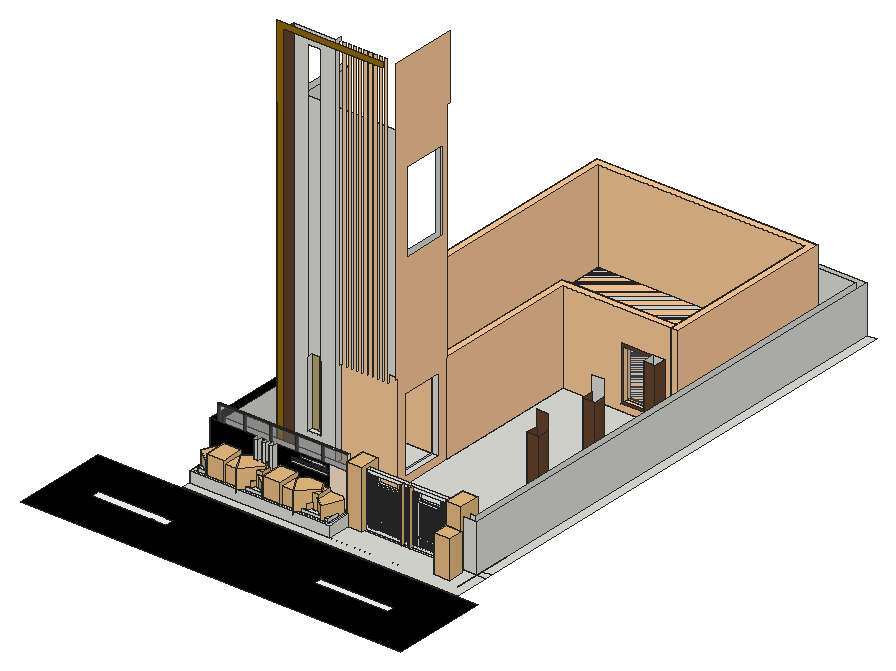
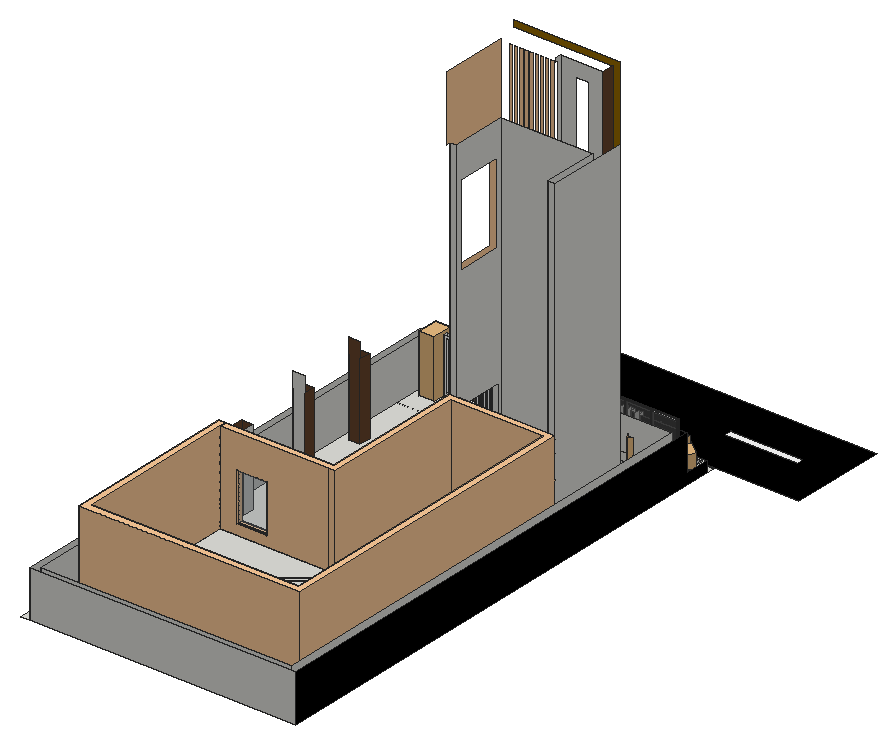
# SketchUp Ruby script. Lengths in inches.
U = 1.inch
M = Sketchup.active_model
def pt(a) = Geom::Point3d.new(a.map { |v| v * U })
def face(e, loops, mat)
  f = e.add_face(loops[0].map { |a| pt(a) })
  loops[1..].each { |l| e.add_face(l.map { |a| pt(a) }).erase! }
  f.material = f.back_material = mat if mat
  f
end
# faces: each face lists its corners as indices into pts; further lists are holes
def faces(e, pts, list, mat = nil) = list.each { |f| face(e, (f[0].is_a?(Array) ? f : [f]).map { |l| l.map { |i| pts[i] } }, mat) }
# xy, xz, yz: faces in a plane at the given z, y or x. An outline is a flat list of corners, or four numbers for a rectangle; further outlines are holes
def ring(l) = l.size == 4 ? [[l[0], l[1]], [l[2], l[1]], [l[2], l[3]], [l[0], l[3]]] : l.each_slice(2).to_a
def flat(e, list, mat, &to3) = list.each { |f| face(e, (f[0].is_a?(Array) ? f : [f]).map { |l| ring(l).map { |u, v| to3.(u, v) } }, mat) }
def xy(e, z, list, mat = nil) = flat(e, list, mat) { |x, y| [x, y, z] }
def xz(e, y, list, mat = nil) = flat(e, list, mat) { |x, z| [x, y, z] }
def yz(e, x, list, mat = nil) = flat(e, list, mat) { |y, z| [x, y, z] }
def lines(e, pts, list) = list.each { |a, b| e.add_line(pt(pts[a]), pt(pts[b])) }
# prism: a flat outline (further loops are holes) pulled along v
def prism(e, loops, v, mat = nil)
  f = face(e, loops, mat); d = Geom::Vector3d.new(v.map { |x| x * U })
  f.pushpull(f.normal.samedirection?(d) ? d.length : -d.length)
end
def box(e, o, s, mat = nil) = prism(e, [[o, [o[0] + s[0], o[1], o[2]], [o[0] + s[0], o[1] + s[1], o[2]], [o[0], o[1] + s[1], o[2]]]], [0, 0, s[2]], mat)
def at(x, y, z, deg = 0) = Geom::Transformation.translation(pt([x, y, z])) * Geom::Transformation.rotation(ORIGIN, Z_AXIS, deg.degrees)
def axes(o, x, y, z) = Geom::Transformation.new([*x, 0, *y, 0, *z, 0, *pt(o).to_a, 1])
def part(name) = M.definitions.add(name)
# library, detail: a bought-in or finely detailed component or shape, given as its bounding box
def library(name, o, s) = part(name).tap { |d| box(d.entities, o, s) }
def detail(e, o, s) = box(e.add_group.entities, o, s)
def put(e, d, t, mat = nil) = e.add_instance(d, t).tap { |i| i.material = mat if mat }
def group(e, t, mat = nil) = e.add_group.tap { |g| g.transformation = t; g.material = mat if mat }.entities
root = M.entities
M.materials.add("Asphalt_06_1K").color = [0, 0, 0]
M.materials.add("C01_Vanilla_Cream").color = [255, 230, 206]
M.materials.add("C02_Golden_Beige").color = [255, 205, 155]
M.materials.add("D07_Ochre_Flame").color = [153, 107, 0]
M.materials.add("Glass_Basic_01").color = [161, 173, 186]
M.materials["Glass_Basic_01"].alpha = 0.25
M.materials.add("Glass_Mirror_01").color = [185, 168, 118]
M.materials.add("M00_Soft_Cloud").color = [255, 255, 255]
M.materials.add("M09_Shadow_Night").color = [0, 0, 0]
M.materials.add("Material__1").color = [95, 70, 46]
M.materials.add("Wood_Veneer_15_1K").color = [103, 69, 45]
M.materials.add("[Color M00]").color = [255, 255, 255]
M.materials.add("[Color_000]").color = [255, 255, 255]
M.materials.add("[Color_C20]").color = [102, 91, 81]
M.materials.add("[Translucent Glass Gray]").color = [128, 128, 128]
M.materials["[Translucent Glass Gray]"].alpha = 0.29
c1 = library("Gate pillar",[0,0,0],[97.06,71.13,326.45])
c2 = library("Group_2",[-1.28,-0.39,0],[21.22,20.51,48.44])
c3 = library("Gate pull handle",[-0.01,0,0],[1.26,2.875,48])
c4 = part("Gate slat")
xy(c4.entities,0,[[0.39,114.16,6.3,114.17]])
xy(c4.entities,0,[[0.39,0,6.3,114.16]],"[Color_C20]")
xy(c4.entities,0.39,[[0.39,0,0.79,114.17],[0.98,0,2.07,114.17],[2.36,0,3.2,114.17],[3.59,0,4.37,114.17],[4.56,0,5.71,114.17],
  [5.91,0,6.3,114.17]],"[Color_C20]")
xy(c4.entities,0.79,[[0.39,0,0.79,114.17],[0.98,0,2.07,114.17],[2.36,0,3.2,114.17],[3.59,0,4.37,114.17],[4.56,0,5.71,114.17],
  [5.91,0,6.3,114.17]],"[Color_C20]")
xy(c4.entities,0.99,[[1.13,0,1.21,114.16],[1.87,0,1.94,114.16],[2.61,0,2.68,114.16],[3.35,0,3.42,114.16],[4.08,0,4.16,114.16],
  [4.82,0,4.9,114.16],[5.5625,0,5.63,114.16],[6.3,0,6.37,114.16]],"[Color_C20]")
xy(c4.entities,1.18,[[0.39,114.16,3.35,114.17],[3.35,114.16,6.3,114.17]])
xy(c4.entities,1.18,[[0.39,0,1.13,114.16],[1.21,0,1.87,114.16],[1.94,0,2.61,114.16],[2.68,0,3.35,114.16],[3.42,0,4.08,114.16],
  [4.16,0,4.82,114.16],[4.9,0,5.5625,114.16],[5.63,0,6.3,114.16]],"[Color_C20]")
xz(c4.entities,0,[[[0.39,0,6.3,0,6.3,0.39,5.91,0.39,5.91,0.79,6.3,0.79,6.3,1.18,5.63,1.18,5.63,0.99,5.5625,0.99,5.5625,1.18,4.9,1.18,4.9,0.99,4.82,0.99,4.82,1.18,4.16,1.18,4.16,0.99,4.08,0.99,4.08,1.18,3.42,1.18,3.42,0.99,3.35,0.99,3.35,1.18,2.68,1.18,2.68,0.99,2.61,0.99,2.61,1.18,1.94,1.18,1.94,0.99,1.87,0.99,1.87,1.18,1.21,1.18,1.21,0.99,1.13,0.99,1.13,1.18,0.39,1.18,0.39,0.79,0.79,0.79,0.79,0.39,0.39,0.39],[4.56,0.39,5.71,0.79],[0.98,0.39,2.07,0.79],[2.36,0.39,3.2,0.79],[3.59,0.39,4.37,0.79]],[6.3,0.99,6.37,1.18]],"[Color_C20]")
xz(c4.entities,114.16,[[1.13,0.99,1.21,1.18],[1.87,0.99,1.94,1.18],[2.61,0.99,2.68,1.18],[3.35,0.99,3.42,1.18],[4.08,0.99,4.16,1.18],
  [4.82,0.99,4.9,1.18],[5.5625,0.99,5.63,1.18]],"[Color_C20]")
xz(c4.entities,114.17,[[[0.39,0,0.39,0.39,0.79,0.39,0.79,0.79,0.39,0.79,0.39,1.18,6.3,1.18,6.3,0.79,5.91,0.79,5.91,0.39,6.3,0.39,6.3,0],[4.56,0.39,5.71,0.79],[0.98,0.39,2.07,0.79],[2.36,0.39,3.2,0.79],[3.59,0.39,4.37,0.79]]],"[Color_C20]")
yz(c4.entities,0.39,[[114.16,0,114.17,0.39],[114.16,0.79,114.17,1.18]])
yz(c4.entities,0.39,[[0,0,114.16,0.39],[0,0.79,114.16,1.18]],"[Color_C20]")
yz(c4.entities,0.79,[[0,0.39,114.17,0.79]],"[Color_C20]")
yz(c4.entities,0.98,[[0,0.39,114.17,0.79]],"[Color_C20]")
yz(c4.entities,1.13,[[0,0.99,114.16,1.18]],"[Color_C20]")
yz(c4.entities,1.21,[[0,0.99,114.16,1.18]],"[Color_C20]")
yz(c4.entities,1.87,[[0,0.99,114.16,1.18]],"[Color_C20]")
yz(c4.entities,1.94,[[0,0.99,114.16,1.18]],"[Color_C20]")
yz(c4.entities,2.07,[[0,0.39,114.17,0.79]],"[Color_C20]")
yz(c4.entities,2.36,[[0,0.39,114.17,0.79]],"[Color_C20]")
yz(c4.entities,2.61,[[0,0.99,114.16,1.18]],"[Color_C20]")
yz(c4.entities,2.68,[[0,0.99,114.16,1.18]],"[Color_C20]")
yz(c4.entities,3.2,[[0,0.39,114.17,0.79]],"[Color_C20]")
yz(c4.entities,3.35,[[0,0.99,114.16,1.18]],"[Color_C20]")
yz(c4.entities,3.42,[[0,0.99,114.16,1.18]],"[Color_C20]")
yz(c4.entities,3.59,[[0,0.39,114.17,0.79]],"[Color_C20]")
yz(c4.entities,4.08,[[0,0.99,114.16,1.18]],"[Color_C20]")
yz(c4.entities,4.16,[[0,0.99,114.16,1.18]],"[Color_C20]")
yz(c4.entities,4.37,[[0,0.39,114.17,0.79]],"[Color_C20]")
yz(c4.entities,4.56,[[0,0.39,114.17,0.79]],"[Color_C20]")
yz(c4.entities,4.82,[[0,0.99,114.16,1.18]],"[Color_C20]")
yz(c4.entities,4.9,[[0,0.99,114.16,1.18]],"[Color_C20]")
yz(c4.entities,5.5625,[[0,0.99,114.16,1.18]],"[Color_C20]")
yz(c4.entities,5.63,[[0,0.99,114.16,1.18]],"[Color_C20]")
yz(c4.entities,5.71,[[0,0.39,114.17,0.79]],"[Color_C20]")
yz(c4.entities,5.91,[[0,0.39,114.17,0.79]],"[Color_C20]")
yz(c4.entities,6.3,[[114.16,0,114.17,0.39],[114.16,0.79,114.17,1.18]])
yz(c4.entities,6.3,[[0,0,114.16,0.39],[0,0.79,114.16,0.99],[0,0.99,114.16,1.18]],"[Color_C20]")
yz(c4.entities,6.37,[[0,0.99,114.16,1.18]],"[Color_C20]")
p = [[0,0,0],[0.39,0,0]]
lines(c4.entities,p,[[0,1]])
c5 = part("Gate infill panel")
put(c5.entities,c4,axes([0,1.18,0],[3.67755,0,0],[0,0,2.40086],[0,-1,0]))
put(c5.entities,c4,axes([21.72,1.18,0],[3.67755,0,0],[0,0,2.40086],[0,-1,0]))
c6 = library("Areca palm plant",[0,0,0],[49.1,36.6,54.46])
c7 = part("W1")
xy(c7.entities,15,[[0,0,2,198]])
xy(c7.entities,102.0625,[[0,0,2,198]],"[Color M00]")
xz(c7.entities,0,[[0,15,2,102.0625]],"[Color M00]")
xz(c7.entities,198,[[0,15,2,102.0625]])
yz(c7.entities,0,[[0.84,16,39.43,101.0625],[40.28,16,78.87,101.0625],[79.71,16,118.3,101.0625],[119.14,16,157.73,101.0625],[158.58,16,197.16,101.0625]])
yz(c7.entities,0,[[[0,15,198,102.0625],[0.84,16,197.16,101.0625]],[39.43,16,40.28,101.0625],[78.87,16,79.71,101.0625],[118.3,16,119.14,101.0625],[157.73,16,158.58,101.0625]],"[Color M00]")
yz(c7.entities,2,[[0.84,16,39.43,101.0625],[40.28,16,78.87,101.0625],[79.71,16,118.3,101.0625],[119.14,16,157.73,101.0625],[158.58,16,197.16,101.0625]])
yz(c7.entities,2,[[[0,15,198,102.0625],[0.84,16,197.16,101.0625]],[39.43,16,40.28,101.0625],[78.87,16,79.71,101.0625],[118.3,16,119.14,101.0625],[157.73,16,158.58,101.0625]],"[Color M00]")
c8 = library("Group\#74",[-84.69,-90.07,-0.36],[176.51,175.13,171.4])
c9 = library("Group20\#1",[-20.81,-17.08,3.79],[39.86,39.43,37.51])
c10 = library("Group\#130",[-7.34,-1.2,0],[38.67,35.81,49.04])
c11 = library("Group38\#2",[14.01,28.44,-23.43],[18.58,18.32,38.89])
c12 = part("PLANTS (1)")
put(c12.entities,c6,axes([38.49,169.84,6.02],[0.45017,-0.56191,0],[0.66137,0.52986,0],[0,0,0.72]))
put(c12.entities,c6,axes([38.49,68.02,6.02],[0.45017,-0.56191,0],[0.66137,0.52986,0],[0,0,0.72]))
put(c12.entities,c7,axes([76.68,11.43,-0.0625],[1,0,0],[0,1.18586,0],[0,0,1]),"[Translucent Glass Gray]")
put(c12.entities,c8,axes([59.61,184.54,5.99],[-0.04961,-0.08593,0],[0.08593,-0.04961,0],[0,0,0.10522]))
put(c12.entities,c8,axes([59.61,204.61,5.99],[-0.04961,-0.08593,0],[0.08593,-0.04961,0],[0,0,0.10522]))
put(c12.entities,c8,axes([59.61,157.29,5.99],[-0.04961,-0.08593,0],[0.08593,-0.04961,0],[0,0,0.10522]))
put(c12.entities,c9,axes([63.65,91.4,4.71],[0,0.85,0],[-0.85,0,0],[0,0,0.85]))
put(c12.entities,c10,axes([69.62,101.34,7.93],[0,0.79,0],[-0.79,0,0],[0,0,0.79]))
put(c12.entities,c11,axes([40.58,10.27,28.11],[0.8848,0,0],[0,0.94674,0],[0,0,0.85826]))
put(c12.entities,c8,axes([59.61,55.48,5.99],[-0.04961,-0.08593,0],[0.08593,-0.04961,0],[0,0,0.10522]))
put(c12.entities,c8,axes([59.61,82.73,5.99],[-0.04961,-0.08593,0],[0.08593,-0.04961,0],[0,0,0.10522]))
put(c12.entities,c8,axes([61.875,132.66,6.01],[-0.08133,-0.14087,0],[0.14087,-0.08133,0],[0,0,0.1725]))
put(c12.entities,c8,axes([59.61,102.79,5.99],[-0.04961,-0.08593,0],[0.08593,-0.04961,0],[0,0,0.10522]))
put(c12.entities,c8,axes([61.875,27.22,6.01],[-0.08133,-0.14087,0],[0.14087,-0.08133,0],[0,0,0.1725]))
put(c12.entities,c8,axes([61.875,234.47,6.01],[-0.08133,-0.14087,0],[0.14087,-0.08133,0],[0,0,0.1725]))
put(c12.entities,c10,axes([69.62,203.15,7.93],[0,0.79,0],[-0.79,0,0],[0,0,0.79]))
put(c12.entities,c9,axes([63.65,193.21,4.71],[0,0.85,0],[-0.85,0,0],[0,0,0.85]))
put(c12.entities,c11,axes([40.58,112.08,28.11],[0.8848,0,0],[0,0.94674,0],[0,0,0.85826]))
g1 = group(c12.entities,at(44.68,11.43,-0.0625))
xy(g1,0,[[0,0,6,234.8],[30,0,36,234.8]])
xy(g1,3,[[6,0,30,234.8]])
xy(g1,7,[[6,5,30,229.8]],"Material__1")
xy(g1,15,[[[0,0,36,234.8],[6,5,30,229.8]]])
xz(g1,0,[[0,0,6,0,6,3,30,3,30,0,36,0,36,15,0,15]])
xz(g1,5,[[6,7,30,15]])
xz(g1,229.8,[[6,7,30,15]])
xz(g1,234.8,[[0,0,0,15,36,15,36,0,30,0,30,3,6,3,6,0]])
yz(g1,0,[[0,0,234.8,15]])
yz(g1,6,[[0,0,234.8,3],[5,7,229.8,15]])
yz(g1,30,[[0,0,234.8,3],[5,7,229.8,15]])
yz(g1,36,[[0,0,234.8,15]])
box(root,[277.79,139.36,-1.58],[179.88,83.23,0.67])
xy(root,-0.91,[[419.54,178.44,419.4375,178.46,419.34,178.53,419.26,178.64,419.2,178.78,419.16,178.94,419.15,179.12,419.16,179.29,419.2,179.45,419.26,179.59,419.34,179.7,419.4375,179.77,419.54,179.79,419.64,179.77,419.73,179.7,419.82,179.59,419.88,179.45,419.92,179.29,419.93,179.12,419.92,178.94,419.88,178.78,419.82,178.64,419.73,178.53,419.64,178.46],[310.61,178.6,310.51,178.625,310.42,178.7,310.34,178.8125,310.27,178.96,310.23,179.14,310.22,179.32,310.23,179.51,310.27,179.6875,310.34,179.84,310.42,179.95,310.51,180.02,310.61,180.05,310.71,180.02,310.81,179.95,310.89,179.84,310.95,179.6875,310.99,179.51,311,179.32,310.99,179.14,310.95,178.96,310.89,178.8125,310.81,178.7,310.71,178.625]])
xy(root,0,[[109.49,127.73,469.49,127.73,469.49,173.01,291.9,173.01,291.9,139.4,109.49,139.4],[112.97,142.89,288.42,169.52],[291.9,173.01,437.93,182.01],[457.3,173.01,469.49,182.01],[[121.46,182.01,437.93,182.01,437.93,183.1,448.27,183.1,448.27,802.53,121.46,802.53],[145.49,236.97,145.49,341.97,283.49,341.97,283.49,260.97,154.49,260.97,154.49,236.97],[422.82,298.73,438.05,313.55],[422.82,390.01,438.05,404.84],[422.82,488.53,438.05,503.35]],
  [457.3,182.01,469.49,809.97],[145.49,236.97,154.49,236.97,154.49,260.97,283.49,260.97,283.49,341.97,274.49,341.97,274.49,269.97,154.73,269.97,154.73,341.97,145.49,341.97],[154.73,269.97,274.49,341.97]])
xy(root,0,[[[0,0,497.19,125.76],[48.65,56.68,144.74,67.55],[338.35,56.68,434.4375,67.55]]],"Asphalt_06_1K")
xy(root,0,[[48.65,56.68,144.74,67.55],[338.35,56.68,434.4375,67.55]],"M00_Soft_Cloud")
xy(root,0.47,[[[308.96,176.2,364.96,181.72],[310.61,178.6,310.71,178.625,310.81,178.7,310.89,178.8125,310.95,178.96,310.99,179.14,311,179.32,310.99,179.51,310.95,179.6875,310.89,179.84,310.81,179.95,310.71,180.02,310.61,180.05,310.51,180.02,310.42,179.95,310.34,179.84,310.27,179.6875,310.23,179.51,310.22,179.32,310.23,179.14,310.27,178.96,310.34,178.8125,310.42,178.7,310.51,178.625]],[[365.1875,176.2,420.13,181.35],[419.54,178.44,419.64,178.46,419.73,178.53,419.82,178.64,419.88,178.78,419.92,178.94,419.93,179.12,419.92,179.29,419.88,179.45,419.82,179.59,419.73,179.7,419.64,179.77,419.54,179.79,419.4375,179.77,419.34,179.7,419.26,179.59,419.2,179.45,419.16,179.29,419.15,179.12,419.16,178.94,419.2,178.78,419.26,178.64,419.34,178.53,419.4375,178.46]]],"[Color_000]")
xy(root,4.04,[[322.85,176.2,324.17,177.12],[324.17,176.2,351.84,177.12],[351.84,176.2,353.16,177.12],[376.99,176.2,378.3125,177.06],[378.3125,176.2,405.98,177.06],
  [405.98,176.2,407.3,177.06]])
xy(root,4.04,[[314.15,176.2,318.5,181.72],[318.5,176.2,322.85,181.72],[353.16,176.2,361.87,177.12],[368.29,176.2,376.99,177.06],[407.3,176.2,411.65,181.35],
  [411.65,176.2,416,181.35],[368.29,177.06,376.99,181.35],[378.3125,177.06,405.98,181.35],[324.17,177.12,351.84,181.72],[353.16,177.12,361.87,181.72]],"[Color_000]")
xy(root,5.39,[[308.96,176.2,311.05,181.72],[419.1,176.2,420.13,181.35]],"[Color_000]")
xy(root,8.97,[[154.49,253.51,209.38,260.97]])
xy(root,9.41,[[274.49,272.89,283.49,328.91]])
xy(root,14.07,[[324.17,176.2,351.84,181.72],[378.3125,176.2,405.98,181.35]],"[Color_000]")
xy(root,14.21,[[[109.49,139.4,291.9,173.01],[112.97,142.89,288.42,169.52]]])
xy(root,15.6,[[324.17,176.2,351.84,181.72],[378.3125,176.2,405.98,181.35]],"[Color_000]")
xy(root,18.94,[[170.97,167.01,176.23,173.01],[181.8125,167.01,187.07,173.01],[191.24,167.01,196.49,173.01]])
xy(root,33.23,[[172.32,253.51,190.09,260.97]])
xy(root,56.18,[[324.17,176.2,351.84,181.72],[378.3125,176.2,405.98,181.35]],"[Color_000]")
xz(root,139.4,[[109.49,0,291.9,14.21]])
xz(root,142.89,[[112.97,0,288.42,14.21]])
xz(root,167.01,[[170.97,18.94,176.23,61.54],[181.8125,18.94,187.07,61.54],[191.24,18.94,196.49,61.54]])
xz(root,169.52,[[112.97,0,288.42,14.21]])
xz(root,173.01,[[437.93,0,457.3,61.54],[215.67,46.96,262.45,48.98],[216.125,51.43,262.66,53.61],[226.02,55.82,262.12,58.61]])
xz(root,173.01,[[264.32,14.21,291.9,61.54]],"C01_Vanilla_Cream")
xz(root,173.01,[[[109.49,14.21,264.32,14.21,264.32,61.54,196.49,61.54,196.49,18.94,191.24,18.94,191.24,61.54,187.07,61.54,187.07,18.94,181.8125,18.94,181.8125,61.54,176.23,61.54,176.23,18.94,170.97,18.94,170.97,61.54,109.49,61.54],[216.125,51.43,262.66,53.61],[226.02,55.82,262.12,58.61],[215.67,46.96,262.45,48.98]]],"M09_Shadow_Night")
xz(root,176.2,[[[308.96,0.47,364.96,0.47,364.96,71.31,311.05,71.31,311.05,5.39,308.96,5.39],[314.15,4.04,361.87,67.74]],[[365.1875,0.47,420.13,0.47,420.13,5.39,419.1,5.39,419.1,71.31,365.1875,71.31],[368.29,4.04,416,67.74]],[322.85,4.04,324.17,14.07],[351.84,4.04,353.16,14.07],[376.99,4.04,378.3125,14.07],
  [405.98,4.04,407.3,14.07],[322.85,14.07,353.16,14.07,353.16,57.7,322.85,57.7,322.85,56.18,351.84,56.18,351.84,15.6,324.17,15.6,324.17,56.18,322.85,56.18],[376.99,14.07,407.3,14.07,407.3,56.18,405.98,56.18,405.98,15.6,378.3125,15.6,378.3125,56.18,407.3,56.18,407.3,57.7,376.99,57.7]],"[Color_000]")
xz(root,181.35,[[[365.1875,0.47,365.1875,71.31,419.1,71.31,419.1,5.39,420.13,5.39,420.13,0.47],[378.3125,15.6,405.98,56.18],[407.3,4.04,416,67.74],[368.29,4.04,376.99,67.74],[378.3125,57.7,405.98,67.74],[378.3125,4.04,405.98,14.07]]],"[Color_000]")
xz(root,181.72,[[[308.96,0.47,308.96,5.39,311.05,5.39,311.05,71.31,364.96,71.31,364.96,0.47],[324.17,15.6,351.84,56.18],[314.15,4.04,322.85,67.74],[353.16,4.04,361.87,67.74],[324.17,57.7,351.84,67.74],[324.17,4.04,351.84,14.07]]],"[Color_000]")
xz(root,182.01,[[121.46,0,291.9,61.54]])
xz(root,183.1,[[437.93,0,448.27,0.87],[437.93,0.87,448.27,61.54]])
xz(root,236.97,[[145.49,0,154.49,0,154.49,503.43,283.49,503.43,283.49,511.11,145.49,511.11]],"D07_Ochre_Flame")
xz(root,253.51,[[[154.49,8.97,209.38,503.43],[172.32,33.23,190.09,485.41]]])
xz(root,260.97,[[154.49,0,283.49,0,283.49,130,273.39,130,273.39,120,270.03,120,270.03,498.95,266.66,498.95,266.66,120,263.3,120,263.3,498.95,259.93,498.95,259.93,120,256.57,120,256.57,498.95,253.2,498.95,253.2,120,249.84,120,249.84,498.95,246.47,498.95,246.47,120,243.11,120,243.11,498.95,239.74,498.95,239.74,120,236.38,120,236.38,498.95,233.01,498.95,233.01,120,229.65,120,229.65,498.95,226.28,498.95,226.28,120,222.92,120,222.92,498.95,219.55,498.95,219.55,120,216.1875,120,216.1875,498.95,212.62,498.95,212.62,120,209.38,120,209.38,8.97,154.49,8.97]],"C02_Golden_Beige")
xz(root,260.97,[[172.32,33.23,181.21,119.26],[181.21,33.23,190.09,119.26]],"Glass_Mirror_01")
xz(root,269.97,[[154.73,0,274.49,414]])
xz(root,272.89,[[274.49,9.41,283.49,106.375]])
xz(root,298.73,[[422.82,0,438.05,99.54]],"Wood_Veneer_15_1K")
xz(root,313.55,[[422.82,0,438.05,120]],"Wood_Veneer_15_1K")
xz(root,328.91,[[274.49,9.41,283.49,106.375]])
xz(root,341.97,[[145.49,0,154.73,414],[274.49,0,283.49,414]])
xz(root,390.01,[[422.82,0,438.05,99.54]],"Wood_Veneer_15_1K")
xz(root,404.84,[[422.82,0,438.05,120]])
xz(root,488.53,[[422.82,0,438.05,99.54]],"Wood_Veneer_15_1K")
xz(root,503.35,[[422.82,0,438.05,99.54]])
xz(root,802.53,[[121.46,0,448.27,61.54]])
xz(root,809.97,[[109.49,0,457.3,61.54]])
yz(root,109.49,[[139.4,0,139.4,14.21,173.01,14.21,173.01,61.54,809.97,61.54,809.97,0]],"M09_Shadow_Night")
yz(root,112.97,[[142.89,0,169.52,14.21]])
yz(root,121.46,[[182.01,0,802.53,61.54]])
yz(root,145.49,[[236.97,0,341.97,414]])
yz(root,154.49,[[236.97,0,260.97,0,260.97,8.97,253.51,8.97,253.51,503.43,236.97,503.43]],"Wood_Veneer_15_1K")
yz(root,154.73,[[269.97,0,341.97,414]])
yz(root,170.97,[[167.01,18.94,173.01,61.54]])
yz(root,172.32,[[253.51,33.23,260.97,119.26]])
yz(root,176.23,[[167.01,18.94,173.01,61.54]])
yz(root,181.8125,[[167.01,18.94,173.01,61.54]])
yz(root,187.07,[[167.01,18.94,173.01,61.54]])
yz(root,190.09,[[253.51,33.23,260.97,119.26]])
yz(root,191.24,[[167.01,18.94,173.01,61.54]])
yz(root,196.49,[[167.01,18.94,173.01,61.54]])
yz(root,209.38,[[253.51,8.97,260.97,8.97,260.97,120,257.97,120,257.97,498.95,260.97,498.95,260.97,503.43,253.51,503.43]])
yz(root,274.49,[[[269.97,0,341.97,414],[275.82,264.75,335.125,370.51],[272.89,9.41,328.91,106.375]]])
yz(root,283.49,[[[260.97,0,341.97,0,341.97,414,346.68,414,346.68,498.95,257.97,498.95,257.97,130,260.97,130],[275.82,264.75,335.125,370.51],[272.89,9.41,328.91,106.375]]],"C02_Golden_Beige")
yz(root,288.42,[[142.89,0,169.52,14.21]])
yz(root,291.9,[[139.4,0,182.01,0,182.01,61.54,173.01,61.54,173.01,14.21,139.4,14.21]])
yz(root,308.96,[[176.2,0.47,181.72,5.39]],"[Color_000]")
yz(root,311.05,[[[176.2,5.39,181.72,71.31],[178.15,57.99,180.23,60.41],[178.15,61.37,180.23,63.7],[178.15,60.52,180.23,61.25]]],"[Color_000]")
yz(root,314.15,[[176.2,4.04,181.72,67.74]],"[Color_000]")
yz(root,322.85,[[176.2,4.04,181.72,14.07],[176.2,14.07,181.72,56.18],[176.2,56.18,181.72,57.7]],"[Color_000]")
yz(root,324.17,[[176.2,4.04,181.72,14.07],[176.2,15.6,181.72,56.18]],"[Color_000]")
yz(root,351.84,[[176.2,4.04,181.72,14.07],[176.2,15.6,181.72,56.18]],"[Color_000]")
yz(root,353.16,[[176.2,4.04,181.72,14.07],[176.2,14.07,181.72,57.7]],"[Color_000]")
yz(root,361.87,[[176.2,4.04,181.72,67.74]],"[Color_000]")
yz(root,364.96,[[176.2,0.47,181.72,71.31]],"[Color_000]")
yz(root,365.1875,[[176.2,0.47,181.35,71.31]],"[Color_000]")
yz(root,368.29,[[176.2,4.04,181.35,67.74]],"[Color_000]")
yz(root,376.99,[[176.2,4.04,181.35,14.07],[176.2,14.07,181.35,57.7]],"[Color_000]")
yz(root,378.3125,[[176.2,4.04,181.35,14.07],[176.2,15.6,181.35,56.18]],"[Color_000]")
yz(root,405.98,[[176.2,4.04,181.35,14.07],[176.2,15.6,181.35,56.18]],"[Color_000]")
yz(root,407.3,[[176.2,4.04,181.35,14.07],[176.2,14.07,181.35,56.18],[176.2,56.18,181.35,57.7]],"[Color_000]")
yz(root,416,[[176.2,4.04,181.35,67.74]],"[Color_000]")
yz(root,419.1,[[[176.2,5.39,181.35,71.31],[178.02,57.99,178.02,60.41,179.96,60.41,179.96,60.52,178.02,60.52,178.02,61.25,179.96,61.25,179.96,57.99],[178.02,61.37,179.96,63.7]]],"[Color_000]")
yz(root,420.13,[[176.2,0.47,181.35,5.39]],"[Color_000]")
yz(root,422.82,[[488.53,0,503.35,99.54]])
yz(root,422.82,[[298.73,0,313.55,99.54],[390.01,0,404.84,99.54]],"Wood_Veneer_15_1K")
yz(root,437.93,[[173.01,0,183.1,61.54]])
yz(root,438.05,[[298.73,0,313.55,99.54],[390.01,0,404.84,99.54],[488.53,0,503.35,99.54]],"Wood_Veneer_15_1K")
yz(root,448.27,[[183.1,0,802.53,61.54]])
yz(root,457.3,[[173.01,0,809.97,61.54]])
p = [[419.54,178.44,0.47],[419.4375,178.46,0.47],[419.4375,178.46,-0.91],[419.54,178.44,-0.91],[419.64,178.46,0.47],[419.64,178.46,-0.91],
  [419.34,178.53,0.47],[419.26,178.64,0.47],[419.26,178.64,-0.91],[419.34,178.53,-0.91],[419.73,178.53,0.47],[419.73,178.53,-0.91],
  [419.82,178.64,0.47],[419.82,178.64,-0.91],[310.51,178.625,0.47],[310.42,178.7,0.47],[310.42,178.7,-0.91],[310.51,178.625,-0.91],
  [310.61,178.6,0.47],[310.61,178.6,-0.91],[310.71,178.625,0.47],[310.71,178.625,-0.91],[310.81,178.7,0.47],[310.81,178.7,-0.91],
  [419.2,178.78,0.47],[419.2,178.78,-0.91],[419.88,178.78,0.47],[419.88,178.78,-0.91],[310.34,178.8125,0.47],[310.34,178.8125,-0.91],
  [310.89,178.8125,0.47],[310.89,178.8125,-0.91],[310.27,178.96,0.47],[310.27,178.96,-0.91],[310.95,178.96,0.47],[310.95,178.96,-0.91],
  [419.16,178.94,0.47],[419.16,178.94,-0.91],[419.92,178.94,0.47],[419.92,178.94,-0.91],[419.15,179.12,0.47],[419.15,179.12,-0.91],
  [419.93,179.12,0.47],[419.93,179.12,-0.91],[310.23,179.14,0.47],[310.23,179.14,-0.91],[310.99,179.14,0.47],[310.99,179.14,-0.91],
  [310.22,179.32,0.47],[310.22,179.32,-0.91],[311,179.32,0.47],[311,179.32,-0.91],[419.16,179.29,0.47],[419.16,179.29,-0.91],
  [419.92,179.29,0.47],[419.92,179.29,-0.91],[310.23,179.51,0.47],[310.23,179.51,-0.91],[310.99,179.51,0.47],[310.99,179.51,-0.91],
  [419.2,179.45,0.47],[419.2,179.45,-0.91],[419.88,179.45,0.47],[419.88,179.45,-0.91],[310.27,179.6875,0.47],[310.27,179.6875,-0.91],
  [310.95,179.6875,0.47],[310.95,179.6875,-0.91],[419.26,179.59,0.47],[419.26,179.59,-0.91],[419.82,179.59,0.47],[419.82,179.59,-0.91],
  [419.34,179.7,0.47],[419.34,179.7,-0.91],[419.73,179.7,0.47],[419.73,179.7,-0.91],[310.34,179.84,0.47],[310.34,179.84,-0.91],
  [310.89,179.84,0.47],[310.89,179.84,-0.91],[419.4375,179.77,0.47],[419.4375,179.77,-0.91],[419.64,179.77,0.47],[419.64,179.77,-0.91],
  [310.42,179.95,0.47],[310.42,179.95,-0.91],[310.81,179.95,0.47],[310.81,179.95,-0.91],[419.54,179.79,0.47],[419.54,179.79,-0.91],
  [310.51,180.02,0.47],[310.51,180.02,-0.91],[310.61,180.05,0.47],[310.61,180.05,-0.91],[310.71,180.02,0.47],[310.71,180.02,-0.91],
  [407.85,177.06,4.04],[407.3,177.06,4.04],[405.97,177.06,58.08],[405.97,177.06,15.6],[322.3,177.12,4.04],[322.85,177.12,4.04],
  [324.18,177.12,58.08],[324.18,177.12,15.6],[364.96,176.2,0.47],[365.1875,176.2,0.47]]
faces(root,p,[[0,1,2,3],[4,0,3,5],[6,7,8,9],[1,6,9,2],[10,4,5,11],[12,10,11,13],[14,15,16,17],[18,14,17,19],
  [20,18,19,21],[22,20,21,23],[7,24,25,8],[26,12,13,27],[15,28,29,16],[30,22,23,31],[28,32,33,29],[34,30,31,35],
  [24,36,37,25],[38,26,27,39],[36,40,41,37],[42,38,39,43],[32,44,45,33],[46,34,35,47],[44,48,49,45],[50,46,47,51],
  [40,52,53,41],[54,42,43,55],[48,56,57,49],[58,50,51,59],[52,60,61,53],[62,54,55,63],[56,64,65,57],[66,58,59,67],
  [60,68,69,61],[70,62,63,71],[68,72,73,69],[74,70,71,75],[64,76,77,65],[78,66,67,79],[72,80,81,73],[82,74,75,83],
  [76,84,85,77],[86,78,79,87],[80,88,89,81],[88,82,83,89],[84,90,91,85],[90,92,93,91],[92,94,95,93],[94,86,87,95]],"[Color_000]")
lines(root,p,[[96,97],[98,99],[100,101],[102,103],[104,105]])
put(root,c1,axes([290.3,169.64,-0.91],[0.20156,0,0],[0,0.374,0],[0,0,0.23238]))
put(root,c1,axes([439.85,169.64,-0.91],[-0.20156,0,0],[0,0.374,0],[0,0,0.23238]))
put(root,c2,at(423.61,146.67,0))
g2 = group(root,at(145.49,341.97,0))
p = [[0,0,0],[0,417,0],[288,417,0],[288,189,0],[138,0,0],[129,198,0],
  [138,198,0],[279,198,0],[279,408,0],[138,189,0],[9,408,0],[9,9,0],
  [129,9,0],[279,189,0]]
lines(g2,p,[[0,1],[1,2],[2,3],[4,0],[5,6],[7,8],[7,6],[4,9],[10,11],[11,12],[9,13],[8,10],
  [12,5]])
g3 = group(root,at(145.49,341.97,0),"C02_Golden_Beige")
xy(g3,0,[[9,9,129,9,129,198,279,198,279,408,9,408]])
xy(g3,12.47,[[217.92,189,257.71,193.5],[217.92,193.5,257.71,198]])
xy(g3,76.47,[[217.92,189,257.71,193.5],[217.92,193.5,257.71,198]])
xy(g3,120,[[0,0,138,0,138,189,279,189,279,198,129,198,129,9,9,9,9,408,279,408,279,189,288,189,288,417,0,417]])
xz(g3,0,[[0,0,138,120]])
xz(g3,9,[[9,0,129,120]])
xz(g3,189,[[[138,0,279,120],[213.92,8.47,261.71,80.47]],[279,0,288,120]])
xz(g3,189,[[[213.92,8.47,261.71,80.47],[217.92,12.47,257.71,76.47]]],"Wood_Veneer_15_1K")
xz(g3,193.5,[[217.92,12.47,257.71,76.47]],"Glass_Basic_01")
xz(g3,198,[[129,0,138,120],[[138,0,279,120],[217.92,12.47,257.71,76.47]]])
xz(g3,408,[[9,0,279,120]])
xz(g3,417,[[0,0,288,120]])
yz(g3,0,[[0,0,417,120]])
yz(g3,9,[[9,0,408,120]])
yz(g3,129,[[9,0,198,120]])
yz(g3,138,[[0,0,189,120]])
yz(g3,217.92,[[189,12.47,193.5,76.47],[193.5,12.47,198,76.47]])
yz(g3,257.71,[[189,12.47,193.5,76.47],[193.5,12.47,198,76.47]])
yz(g3,279,[[189,0,198,120],[198,0,408,120]])
yz(g3,288,[[189,0,417,120]])
put(root,c3,axes([370.96,171.71,0.75],[-0.86672,0,0],[0,1.56297,0],[0,0,1.46989]))
put(root,c3,axes([359.2,171.39,0.75],[0.86672,0,0],[0,1.67487,0],[0,0,1.46989]))
put(root,c5,axes([378.3125,177.06,3.7],[0,0,0.23699],[0,0.34901,0],[0.10093,0,0]))
put(root,c5,axes([351.84,177.12,3.7],[0,0,0.23699],[0,0.374,0],[-0.10093,0,0]))
put(root,c4,axes([416.35,177.47,4.04],[-0.74126,0,0],[0,0,0.55792],[0,-0.34901,0]))
put(root,c4,axes([411.97,177.47,4.04],[-0.74126,0,0],[0,0,0.55792],[0,-0.34901,0]))
put(root,c4,axes([372.95,177.47,4.04],[-0.74126,0,0],[0,0,0.55792],[0,-0.34901,0]))
put(root,c4,axes([377.33,177.47,4.04],[-0.74126,0,0],[0,0,0.55792],[0,-0.34901,0]))
put(root,c4,axes([313.81,177.56,4.04],[0.74126,0,0],[0,0,0.55792],[0,-0.374,0]))
put(root,c4,axes([318.18,177.56,4.04],[0.74126,0,0],[0,0,0.55792],[0,-0.374,0]))
put(root,c4,axes([352.82,177.56,4.04],[0.74126,0,0],[0,0,0.55792],[0,-0.374,0]))
put(root,c4,axes([357.2,177.56,4.04],[0.74126,0,0],[0,0,0.55792],[0,-0.374,0]))
put(root,c12,axes([293.6,100.07,5.95],[0,1.02194,0],[-0.72563,0,0],[0,0,0.7056]))
put(root,c5,axes([378.31,177.06,15.47],[0,0,0.23236],[0,0.34901,0],[0.10093,0,0]))
put(root,c5,axes([351.84,177.12,15.47],[0,0,0.23236],[0,0.374,0],[-0.10093,0,0]))
put(root,c5,axes([378.31,177.06,25.57],[0,0,0.23236],[0,0.34901,0],[0.10093,0,0]))
put(root,c5,axes([351.84,177.12,25.57],[0,0,0.23236],[0,0.374,0],[-0.10093,0,0]))
put(root,c5,axes([378.3125,177.06,35.66],[0,0,0.23236],[0,0.34901,0],[0.10093,0,0]))
put(root,c5,axes([351.84,177.12,35.66],[0,0,0.23236],[0,0.374,0],[-0.10093,0,0]))
put(root,c5,axes([378.3125,177.06,45.75],[0,0,0.23236],[0,0.34901,0],[0.10093,0,0]))
put(root,c5,axes([351.84,177.12,45.75],[0,0,0.23236],[0,0.374,0],[-0.10093,0,0]))
